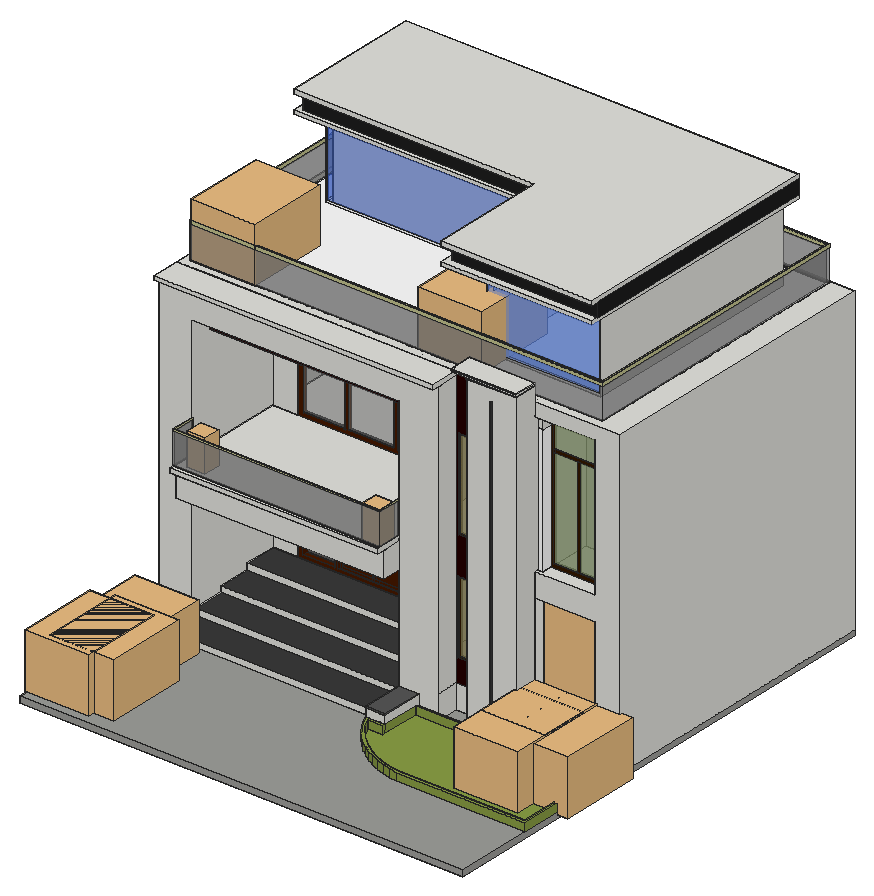
# SketchUp Ruby script. Lengths in inches.
U = 1.inch
M = Sketchup.active_model
def pt(a) = Geom::Point3d.new(a.map { |v| v * U })
def face(e, loops, mat)
  f = e.add_face(loops[0].map { |a| pt(a) })
  loops[1..].each { |l| e.add_face(l.map { |a| pt(a) }).erase! }
  f.material = f.back_material = mat if mat
  f
end
# faces: each face lists its corners as indices into pts; further lists are holes
def faces(e, pts, list, mat = nil) = list.each { |f| face(e, (f[0].is_a?(Array) ? f : [f]).map { |l| l.map { |i| pts[i] } }, mat) }
# xy, xz, yz: faces in a plane at the given z, y or x. An outline is a flat list of corners, or four numbers for a rectangle; further outlines are holes
def ring(l) = l.size == 4 ? [[l[0], l[1]], [l[2], l[1]], [l[2], l[3]], [l[0], l[3]]] : l.each_slice(2).to_a
def flat(e, list, mat, &to3) = list.each { |f| face(e, (f[0].is_a?(Array) ? f : [f]).map { |l| ring(l).map { |u, v| to3.(u, v) } }, mat) }
def xy(e, z, list, mat = nil) = flat(e, list, mat) { |x, y| [x, y, z] }
def xz(e, y, list, mat = nil) = flat(e, list, mat) { |x, z| [x, y, z] }
def yz(e, x, list, mat = nil) = flat(e, list, mat) { |y, z| [x, y, z] }
def lines(e, pts, list) = list.each { |a, b| e.add_line(pt(pts[a]), pt(pts[b])) }
# prism: a flat outline (further loops are holes) pulled along v
def prism(e, loops, v, mat = nil)
  f = face(e, loops, mat); d = Geom::Vector3d.new(v.map { |x| x * U })
  f.pushpull(f.normal.samedirection?(d) ? d.length : -d.length)
end
def box(e, o, s, mat = nil) = prism(e, [[o, [o[0] + s[0], o[1], o[2]], [o[0] + s[0], o[1] + s[1], o[2]], [o[0], o[1] + s[1], o[2]]]], [0, 0, s[2]], mat)
def at(x, y, z, deg = 0) = Geom::Transformation.translation(pt([x, y, z])) * Geom::Transformation.rotation(ORIGIN, Z_AXIS, deg.degrees)
def axes(o, x, y, z) = Geom::Transformation.new([*x, 0, *y, 0, *z, 0, *pt(o).to_a, 1])
def part(name) = M.definitions.add(name)
# library, detail: a bought-in or finely detailed component or shape, given as its bounding box
def library(name, o, s) = part(name).tap { |d| box(d.entities, o, s) }
def detail(e, o, s) = box(e.add_group.entities, o, s)
def put(e, d, t, mat = nil) = e.add_instance(d, t).tap { |i| i.material = mat if mat }
def group(e, t, mat = nil) = e.add_group.tap { |g| g.transformation = t; g.material = mat if mat }.entities
root = M.entities
M.materials.add("[Color A08]").color = [37, 0, 0]
M.materials.add("[Color B08]").color = [71, 25, 0]
M.materials.add("[Color B08]1").color = [52, 25, 0]
M.materials.add("[Color M00]").color = [255, 255, 255]
M.materials.add("[Color M06]").color = [86, 86, 86]
M.materials.add("[Color M07]").color = [58, 58, 58]
M.materials.add("[Color M08]").color = [30, 30, 30]
M.materials.add("[Concrete Block 8x8 Gray]").color = [157, 158, 154]
M.materials.add("[Grass Light Green]").color = [138, 158, 69]
M.materials.add("[Metal Corrugated Shiny]").color = [193, 193, 151]
M.materials.add("[Metal Corrugated Shiny]1").color = [193, 193, 141]
M.materials.add("[Translucent Glass Corrugated]").color = [141, 132, 85]
M.materials["[Translucent Glass Corrugated]"].alpha = 0.8
M.materials.add("[Translucent Glass Corrugated]1").color = [141, 158, 115]
M.materials["[Translucent Glass Corrugated]1"].alpha = 0.8
M.materials.add("[Translucent Glass Gray]").color = [128, 128, 128]
M.materials["[Translucent Glass Gray]"].alpha = 0.5
M.materials.add("[Translucent Glass Safety]").color = [100, 143, 244]
M.materials["[Translucent Glass Safety]"].alpha = 0.5
M.materials.add("[Translucent Glass Safety]1").color = [69, 115, 244]
M.materials["[Translucent Glass Safety]1"].alpha = 0.5
c1 = library("ARTIFICIAL PLANTS",[20.77,3.52,-2.22],[96.42,122.82,82.56])
c2 = library("Plant",[12.07,-11.84,0],[27.54,27.97,38.79])
c3 = part("Group\#3")
xy(c3.entities,0,[[0,0,37.8125,3.1875]],"[Color B08]1")
xy(c3.entities,2.15,[[2.15,0,35.67,0.6875],[2.15,0.6875,35.67,3.1875]],"[Color B08]1")
xy(c3.entities,107.17,[[2.15,0,35.67,0.6875],[2.15,0.6875,35.67,3.1875]],"[Color B08]1")
xy(c3.entities,109.3125,[[0,0,37.8125,3.1875]],"[Color B08]1")
xz(c3.entities,0,[[[0,0,37.8125,109.3125],[2.15,2.15,35.67,107.17]]],"[Color B08]1")
xz(c3.entities,0.6875,[[2.15,2.15,35.67,107.17]],"[Translucent Glass Corrugated]")
xz(c3.entities,3.1875,[[[0,0,37.8125,109.3125],[2.15,2.15,35.67,107.17]]],"[Color B08]1")
yz(c3.entities,0,[[0,0,3.1875,109.3125]],"[Color B08]1")
yz(c3.entities,2.15,[[0,2.15,0.6875,107.17],[0.6875,2.15,3.1875,107.17]],"[Color B08]1")
yz(c3.entities,35.67,[[0,2.15,0.6875,107.17],[0.6875,2.15,3.1875,107.17]],"[Color B08]1")
yz(c3.entities,37.8125,[[0,0,3.1875,109.3125]],"[Color B08]1")
c4 = library("Group\#4",[0,0,0],[79.3125,7.3125,150.8125])
xy(root,0,[[0,0,667.75,739.0625]])
xy(root,9,[[24.41,199.0625,48.8125,262.25],[362.125,199.0625,391.71,262.25],[0,262.25,48.8125,295.75],[362.125,262.25,421.3,295.75],[[0,295.75,0,739.0625,667.75,739.0625,667.75,295.75,539.36,295.75,539.36,301.75,547.4375,301.75,547.4375,730.0625,366.0625,730.0625,366.0625,415.1875,48.8125,415.1875,48.8125,295.75],[48.8125,421.1875,362.125,730.0625],[553.4375,301.75,630.8125,730.0625]],
  [362.125,295.75,463.53,301.75],[362.125,301.75,366.0625,415.1875],[366.0625,301.75,547.4375,730.0625],[553.4375,301.75,630.8125,730.0625],[48.8125,421.1875,362.125,730.0625]])
xy(root,9,[[500.61,259.1875,502.54,262.25]],"[Color M07]")
xy(root,9,[[0,0,667.75,0,667.75,117.6,474.66,117.6,462.59,119.14,450.71,121.76,439.11,125.45,427.9,130.18,417.16,135.91,406.99,142.59,397.47,150.16,388.68,158.57,380.68,167.75,373.55,177.61,367.35,188.07,362.125,199.0625,362.125,415.1875,48.8125,415.1875,48.8125,199.0625,24.41,199.0625,24.41,262.25,0,262.25],[391.71,259.1875,500.61,259.1875,500.61,262.25,463.53,262.25,463.53,295.75,421.3,295.75,421.3,262.25,391.71,262.25]],"[Concrete Block 8x8 Gray]")
xy(root,9,[[474.66,117.6,462.59,119.14,450.71,121.76,439.11,125.45,427.9,130.18,417.16,135.91,406.99,142.59,397.47,150.16,388.68,158.57,380.68,167.75,373.55,177.61,367.35,188.07,362.125,199.0625,391.71,199.0625,391.71,195.14,368.33,195.14,370.82,189.92,376.84,179.76,383.76,170.1875,391.52,161.28,400.05,153.12,409.3,145.77,419.17,139.29,429.59,133.73,440.47,129.14,451.73,125.55,463.26,123.01,474.91,121.53,663.83,121.53,663.83,292.2,539.36,292.2,539.36,295.75,667.75,295.75,667.75,117.6],[474.91,121.53,663.83,121.53,663.83,292.2,541.86,292.2,541.86,256.08,391.71,256.08,391.71,195.14,368.33,195.14,370.82,189.92,376.84,179.76,383.76,170.1875,391.52,161.28,400.05,153.12,409.3,145.77,419.17,139.29,429.59,133.73,440.47,129.14,451.73,125.55,463.26,123.01],[391.71,256.08,391.71,259.1875,502.54,259.1875,502.54,262.25,541.86,262.25,541.86,256.08]],"[Grass Light Green]")
xy(root,21,[[474.66,117.6,667.75,117.6,667.75,295.75,539.36,295.75,539.36,262.25,502.54,262.25,502.54,259.1875,391.71,259.1875,391.71,256.08,541.86,256.08,541.86,292.2,663.83,292.2,663.83,121.53,474.91,121.53,463.26,123.01,451.73,125.55,440.47,129.14,429.59,133.73,419.17,139.29,409.3,145.77,400.05,153.12,391.52,161.28,383.76,170.1875,376.84,179.76,370.82,189.92,368.33,195.14,391.71,195.14,391.71,199.0625,362.125,199.0625,367.35,188.07,373.55,177.61,380.68,167.75,388.68,158.57,397.47,150.16,406.99,142.59,417.16,135.91,427.9,130.18,439.11,125.45,450.71,121.76,462.59,119.14]],"[Grass Light Green]")
xy(root,33,[[24.41,199.0625,48.8125,262.25],[362.125,199.0625,391.71,262.25]])
xy(root,35,[[362.125,199.0625,391.71,262.25]],"[Color M06]")
xy(root,35.25,[[24.41,199.0625,48.8125,262.25]],"[Color M06]")
xy(root,45,[[547.4375,295.75,547.4375,303.1875,553.4375,303.1875,553.4375,301.75,553.875,301.75,553.875,295.75],[553.875,295.75,630.8125,301.75],[553.4375,301.75,553.875,730.0625],[547.4375,303.1875,553.4375,730.0625],[86.78,415.1875,319.35,421.1875]])
xy(root,79.74,[[424.46,295.75,460.15,301.75]])
xy(root,182,[[86.78,415.1875,319.35,421.1875]])
xy(root,190.99,[[424.46,295.75,460.15,301.75]])
xy(root,191.8125,[[48.8125,232.8125,362.125,415.1875]])
xy(root,201,[[547.4375,295.75,547.4375,303.1875,553.4375,303.1875,553.4375,301.75,553.875,301.75,553.875,295.75],[362.125,301.75,366.0625,415.1875],[553.4375,301.75,553.875,381.8125],[547.4375,303.1875,553.4375,730.0625]])
xy(root,201,[[553.875,295.75,630.8125,381.8125]],"[Color M00]")
xy(root,211.75,[[553.4375,381.8125,630.8125,730.0625]])
xy(root,227.875,[[48.8125,421.1875,362.125,730.0625]])
xy(root,230.8125,[[48.8125,222.0625,362.125,232.8125],[48.8125,232.8125,48.8125,415.1875,86.78,415.1875,86.78,421.1875,319.35,421.1875,319.35,415.1875,362.125,415.1875,362.125,232.8125]])
xy(root,231,[[366.0625,301.75,547.4375,730.0625]])
xy(root,237,[[48.8125,222.0625,362.125,226.625],[48.8125,226.625,48.8125,262.25,50.625,262.25,50.625,228.625,360.31,228.625,360.31,262.25,362.125,262.25,362.125,226.625],[50.625,228.625,360.31,228.625,360.31,262.25,362.125,262.25,362.125,415.1875,319.35,415.1875,319.35,421.1875,86.78,421.1875,86.78,415.1875,48.8125,415.1875,48.8125,262.25,50.625,262.25],[539.36,295.75,539.36,301.75,547.4375,301.75,547.4375,316.75,630.8125,316.75,630.8125,295.75],[362.125,301.75,366.0625,415.1875],
  [366.0625,301.75,547.4375,730.0625],[547.4375,320.84,630.8125,381.8125],[553.4375,381.8125,630.8125,730.0625],[48.8125,421.1875,362.125,730.0625]])
xy(root,237,[[547.4375,316.75,630.8125,320.84]],"[Color B08]1")
xy(root,242.04,[[551.26,316.75,587.21,318.46],[587.21,316.75,590.4375,318.46],[590.4375,316.75,626.99,318.46],[551.26,318.46,587.21,320.84],[587.21,318.46,590.4375,320.84],
  [590.4375,318.46,626.99,320.84]],"[Color B08]1")
xy(root,246,[[425.47,295.75,460.78,301.75]])
xy(root,285,[[48.8125,226.625,48.8125,262.25,50.625,262.25,50.625,228.625,360.31,228.625,360.31,262.25,362.125,262.25,362.125,226.625]])
xy(root,287.0625,[[48.8125,226.625,362.125,226.625,362.125,262.25,360.31,262.25,360.31,228.625,50.625,228.625,50.625,262.25,48.8125,262.25]],"[Metal Corrugated Shiny]1")
xy(root,374,[[86.78,415.1875,319.35,421.1875]])
xy(root,384.44,[[425.47,295.75,460.78,301.75]])
xy(root,393,[[362.125,301.75,366.0625,415.1875]])
xy(root,393,[[48.8125,295.75,362.125,415.1875]],"[Color M07]")
xy(root,419.72,[[48.8125,262.25,362.125,295.75]])
xy(root,429,[[366.0625,301.75,547.375,301.75,547.375,336.875,547.4375,336.875,547.4375,730.0625,366.0625,730.0625],[547.375,301.75,547.4375,332.6875],[547.4375,301.75,547.875,332.6875],[547.375,332.6875,547.4375,336.875],[547.4375,381.8125,553.4375,730.0625],
  [553.4375,381.8125,630.8125,730.0625]])
xy(root,429,[[547.4375,332.6875,630.8125,381.8125]],"[Color M00]")
xy(root,441.39,[[551.26,316.75,626.99,318.46],[551.26,318.46,626.99,320.84]],"[Color B08]1")
xy(root,446.4375,[[539.36,295.75,547.875,301.75],[547.875,295.75,630.8125,316.75],[366.0625,301.75,366.0625,730.0625,630.8125,730.0625,630.8125,336.875,547.375,336.875,547.375,301.75],[547.375,301.75,547.875,301.75,547.875,316.75,547.4375,316.75,547.4375,320.84,547.875,320.84,547.875,332.6875,630.8125,332.6875,630.8125,336.875,547.375,336.875],[547.4375,316.75,547.875,320.84],
  [547.875,320.84,630.8125,332.6875]])
xy(root,446.4375,[[547.875,316.75,630.8125,320.84]],"[Color B08]1")
xy(root,460.0625,[[0,252.125,421.3,262.25],[0,262.25,421.3,295.75]])
xy(root,466.375,[[0,252.125,421.3,295.75],[[0,295.75,667.75,739.0625],[9.3125,307.9375,632.75,735.0625]],[[9.3125,307.9375,632.75,735.0625],[11.3125,309.9375,630.75,733.0625]],[[420.125,354.47,420.125,517.125,48.125,517.125,48.125,696.4375,593.125,696.4375,593.125,354.47],[426.125,360.47,587.125,360.47,587.125,690.4375,54.125,690.4375,54.125,523.125,426.125,523.125]],[426.125,360.47,587.125,360.47,587.125,690.4375,54.125,690.4375,54.125,523.125,426.125,523.125]])
xy(root,466.375,[[[11.3125,309.9375,630.75,733.0625],[420.125,354.47,593.125,354.47,593.125,696.4375,48.125,696.4375,48.125,517.125,420.125,517.125]]],"[Color M00]")
xy(root,467.84,[[500.61,259.1875,502.54,262.25]],"[Color M07]")
xy(root,486.125,[[463.53,261.625,539.36,262.25],[463.53,262.25,539.36,295.75]])
xy(root,488.1875,[[442.91,260.8125,463.53,295.75],[463.53,260.8125,539.36,261.625],[463.53,261.625,539.36,295.75]])
xy(root,490.625,[[441.16,260.0625,442.91,295.75],[442.91,260.0625,539.36,260.8125],[442.91,260.8125,539.36,295.75]])
xy(root,492.0625,[[441.16,260.0625,539.36,295.75]])
xy(root,514.375,[[[9.3125,307.9375,632.75,735.0625],[11.3125,309.9375,630.75,733.0625]]])
xy(root,519.75,[[[9.3125,307.9375,632.75,735.0625],[11.3125,309.9375,630.75,733.0625]]],"[Metal Corrugated Shiny]1")
xy(root,580.375,[[426.125,360.47,426.125,523.125,54.125,523.125,54.125,690.4375,587.125,690.4375,587.125,360.47]])
xy(root,586.375,[[381.75,315.41,381.75,492.1875,18.75,492.1875,18.75,704.25,48.125,704.25,48.125,517.125,420.125,517.125,420.125,354.47,593.125,354.47,593.125,696.4375,63,696.4375,63,704.25,610.625,704.25,610.625,315.41],[420.125,354.47,426.125,508.125],[426.125,354.47,593.125,360.47],[426.125,360.47,426.125,523.125,54.125,523.125,54.125,690.4375,587.125,690.4375,587.125,360.47],[587.125,360.47,593.125,690.4375],
  [420.125,508.125,426.125,508.125,426.125,523.125,54.125,523.125,54.125,517.125,420.125,517.125],[48.125,517.125,54.125,696.4375],[54.125,690.4375,63,696.4375],[63,690.4375,593.125,696.4375],[48.125,696.4375,54.125,704.25],
  [54.125,696.4375,63,704.25]])
xy(root,591.75,[[381.75,315.41,610.625,315.41,610.625,326.35,390.1875,326.35,390.1875,492.1875,381.75,492.1875],[390.1875,326.35,610.625,326.35,610.625,704.25,63,704.25,63,696.4375,593.125,696.4375,593.125,354.47,420.125,354.47,420.125,517.125,48.125,517.125,48.125,704.25,28.5625,704.25,28.5625,498.4375,390.1875,498.4375],[420.125,354.47,593.125,354.47,593.125,696.4375,63,696.4375,63,704.25,48.125,704.25,48.125,517.125,420.125,517.125],[18.75,492.1875,390.1875,492.1875,390.1875,498.4375,28.5625,498.4375,28.5625,704.25,18.75,704.25]])
xy(root,612.75,[[381.75,315.41,381.75,492.1875,18.75,492.1875,18.75,704.25,28.5625,704.25,28.5625,498.4375,390.1875,498.4375,390.1875,326.35,610.625,326.35,610.625,315.41]])
xy(root,619.25,[[381.75,315.41,610.625,315.41,610.625,704.25,18.75,704.25,18.75,492.1875,381.75,492.1875]])
xz(root,0,[[0,0,667.75,9]],"[Concrete Block 8x8 Gray]")
xz(root,117.6,[[474.66,9,667.75,21]],"[Grass Light Green]")
xz(root,121.53,[[474.91,9,663.83,21]],"[Grass Light Green]")
xz(root,195.14,[[368.33,9,391.71,21]],"[Grass Light Green]")
xz(root,199.0625,[[24.41,9,48.8125,33],[362.125,21,391.71,33]])
xz(root,199.0625,[[24.41,33,48.8125,35.25],[362.125,33,391.71,35]],"[Color M06]")
xz(root,199.0625,[[362.125,9,391.71,21]],"[Grass Light Green]")
xz(root,222.0625,[[48.8125,230.8125,362.125,237]])
xz(root,226.625,[[48.8125,285,362.125,287.0625]],"[Metal Corrugated Shiny]1")
xz(root,226.625,[[48.8125,237,362.125,285]],"[Translucent Glass Gray]")
xz(root,228.625,[[50.625,285,360.31,287.0625]],"[Metal Corrugated Shiny]1")
xz(root,228.625,[[50.625,237,360.31,285]],"[Translucent Glass Gray]")
xz(root,232.8125,[[48.8125,191.8125,362.125,230.8125]])
xz(root,252.125,[[0,460.0625,421.3,466.375]])
xz(root,256.08,[[391.71,9,541.86,21]],"[Grass Light Green]")
xz(root,259.1875,[[500.61,9,502.54,21],[500.61,21,502.54,467.84]],"[Color M07]")
xz(root,259.1875,[[391.71,9,500.61,21]],"[Grass Light Green]")
xz(root,260.0625,[[441.16,490.625,539.36,492.0625]])
xz(root,260.8125,[[442.91,488.1875,539.36,490.625]])
xz(root,261.625,[[463.53,486.125,539.36,488.1875]])
xz(root,262.25,[[0,9,24.41,9,24.41,35.25,48.8125,35.25,48.8125,419.72,362.125,419.72,362.125,35,391.71,35,391.71,9,421.3,9,421.3,460.0625,0,460.0625],[24.41,9,48.8125,33],[362.125,9,391.71,33],[463.53,9,500.61,9,500.61,467.84,502.54,467.84,502.54,21,539.36,21,539.36,486.125,463.53,486.125],[24.41,33,48.8125,35.25],
  [362.125,33,391.71,35],[48.8125,237,50.625,285],[360.31,237,362.125,285],[48.8125,285,50.625,287.0625],[360.31,285,362.125,287.0625]])
xz(root,262.25,[[500.61,9,502.54,467.84]],"[Color M07]")
xz(root,292.2,[[541.86,9,663.83,21]],"[Grass Light Green]")
xz(root,295.75,[[421.3,9,463.53,45],[539.36,21,667.75,21,667.75,466.375,539.36,466.375,539.36,446.4375,630.8125,446.4375,630.8125,237,539.36,237,539.36,201,630.8125,201,630.8125,45,539.36,45],[539.36,45,553.875,201],[48.8125,419.72,362.125,460.0625],[0,460.0625,48.8125,466.375],
  [48.8125,460.0625,362.125,466.375],[362.125,460.0625,421.3,466.375],[463.53,466.375,539.36,486.125],[463.53,486.125,539.36,488.1875],[442.91,488.1875,539.36,490.625],
  [441.16,490.625,539.36,492.0625]])
xz(root,295.75,[[[421.3,45,463.53,466.375],[425.47,246,460.78,384.44],[424.46,79.74,460.15,190.99]],[48.8125,393,362.125,419.72]],"[Color A08]")
xz(root,301.75,[[[366.0625,9,463.53,231],[424.46,79.74,460.15,190.99]],[463.53,9,539.36,45],[539.36,9,547.4375,45],[553.4375,9,630.8125,45],[463.53,45,539.36,201],
  [539.36,45,547.4375,201],[553.4375,45,553.875,201],[362.125,201,366.0625,237],[463.53,201,539.36,231],[539.36,201,547.4375,231],
  [366.0625,231,463.53,237],[463.53,231,539.36,237],[539.36,231,547.4375,237],[[366.0625,237,539.36,429],[425.47,246,460.78,384.44]],[366.0625,429,539.36,446.4375],
  [539.36,429,547.875,446.4375],[463.53,446.4375,539.36,460.0625]])
xz(root,301.75,[[539.36,237,547.4375,429]],"[Color M00]")
xz(root,303.1875,[[547.4375,45,553.4375,201]])
xz(root,307.9375,[[9.3125,514.375,632.75,519.75]],"[Metal Corrugated Shiny]1")
xz(root,307.9375,[[9.3125,466.375,632.75,514.375]],"[Translucent Glass Gray]")
xz(root,309.9375,[[11.3125,514.375,630.75,519.75]],"[Metal Corrugated Shiny]1")
xz(root,309.9375,[[11.3125,466.375,630.75,514.375]],"[Translucent Glass Gray]")
xz(root,315.41,[[381.75,586.375,610.625,591.75],[381.75,612.75,610.625,619.25]])
xz(root,316.75,[[[547.4375,237,630.8125,446.4375],[551.26,242.04,626.99,441.39]]],"[Color B08]1")
xz(root,318.46,[[587.21,242.04,590.4375,391.43],[551.26,391.43,626.99,396.74]],"[Color B08]1")
xz(root,318.46,[[551.26,242.04,587.21,391.43],[590.4375,242.04,626.99,391.43],[551.26,396.74,626.99,441.39]],"[Translucent Glass Corrugated]1")
xz(root,320.84,[[[547.4375,237,630.8125,446.4375],[551.26,242.04,626.99,441.39]]],"[Color B08]1")
xz(root,326.35,[[390.1875,591.75,610.625,612.75]],"[Color M08]")
xz(root,332.6875,[[547.875,429,630.8125,446.4375]])
xz(root,354.47,[[420.125,586.375,426.125,591.75],[426.125,586.375,593.125,591.75]])
xz(root,354.47,[[[420.125,466.375,593.125,586.375],[422.51,468.76,590.74,583.99]]],"[Color M00]")
xz(root,354.47,[[422.51,468.76,590.74,583.99]],"[Translucent Glass Safety]")
xz(root,360.47,[[426.125,580.375,587.125,586.375]])
xz(root,360.47,[[426.125,466.375,587.125,580.375]],"[Translucent Glass Safety]")
xz(root,381.8125,[[553.4375,201,630.8125,211.75],[553.4375,211.75,630.8125,237],[547.4375,237,630.8125,429]])
xz(root,415.1875,[[48.8125,9,362.125,45],[362.125,9,366.0625,45],[48.8125,45,86.78,45,86.78,182,319.35,182,319.35,45,362.125,45,362.125,191.8125,48.8125,191.8125],[362.125,45,366.0625,201],[48.8125,230.8125,86.78,237],
  [319.35,230.8125,362.125,237],[48.8125,237,86.78,237,86.78,374,319.35,374,319.35,237,362.125,237,362.125,393,48.8125,393],[362.125,237,366.0625,393]])
xz(root,421.1875,[[48.8125,9,362.125,45],[48.8125,45,48.8125,201,362.125,201,362.125,45,319.35,45,319.35,182,86.78,182,86.78,45],[48.8125,201,362.125,227.875],[48.8125,227.875,86.78,237],[86.78,227.875,319.35,230.8125],
  [319.35,227.875,328.9375,237],[328.9375,227.875,350.5,237],[350.5,227.875,362.125,237],[86.78,230.8125,319.35,237],[48.8125,237,48.8125,393,362.125,393,362.125,237,319.35,237,319.35,374,86.78,374,86.78,237],
  [48.8125,393,362.125,429]])
xz(root,492.1875,[[18.75,586.375,381.75,591.75],[18.75,612.75,381.75,619.25]])
xz(root,498.4375,[[28.5625,591.75,390.1875,612.75]],"[Color M08]")
xz(root,517.125,[[48.125,586.375,54.125,591.75],[54.125,586.375,420.125,591.75]])
xz(root,517.125,[[[48.125,466.375,420.125,586.375],[50.82,469.07,417.43,583.68]]],"[Color M00]")
xz(root,517.125,[[50.82,469.07,417.43,583.68]],"[Translucent Glass Safety]1")
xz(root,523.125,[[54.125,466.375,426.125,580.375],[54.125,580.375,426.125,586.375]])
xz(root,690.4375,[[54.125,466.375,587.125,580.375],[54.125,580.375,63,586.375],[63,580.375,587.125,586.375]])
xz(root,696.4375,[[48.125,466.375,593.125,586.375],[63,586.375,593.125,591.75]])
xz(root,704.25,[[18.75,586.375,610.625,591.75],[18.75,612.75,610.625,619.25]])
xz(root,704.25,[[28.5625,591.75,610.625,612.75]],"[Color M08]")
xz(root,730.0625,[[48.8125,9,362.125,45],[366.0625,9,547.4375,45],[553.4375,9,630.8125,45],[48.8125,45,362.125,201],[366.0625,45,547.4375,201],
  [547.4375,45,553.4375,201],[553.4375,45,553.875,201],[553.875,45,630.8125,201],[48.8125,201,362.125,227.875],[366.0625,201,547.4375,231],
  [547.4375,201,553.4375,429],[553.4375,201,630.8125,211.75],[553.4375,211.75,561.3125,237],[561.3125,211.75,573.8125,237],[573.8125,211.75,630.8125,237],
  [48.8125,227.875,362.125,237],[366.0625,231,547.4375,237],[48.8125,237,362.125,393],[366.0625,237,547.4375,393],[553.4375,237,630.8125,393],
  [48.8125,393,362.125,429],[366.0625,393,547.4375,429],[553.4375,393,630.8125,429],[366.0625,429,547.4375,446.4375],[547.4375,429,553.4375,446.4375],
  [553.4375,429,630.8125,446.4375]])
xz(root,733.0625,[[11.3125,514.375,630.75,519.75]],"[Metal Corrugated Shiny]1")
xz(root,733.0625,[[11.3125,466.375,630.75,514.375]],"[Translucent Glass Gray]")
xz(root,735.0625,[[9.3125,514.375,632.75,519.75]],"[Metal Corrugated Shiny]1")
xz(root,735.0625,[[9.3125,466.375,632.75,514.375]],"[Translucent Glass Gray]")
xz(root,739.0625,[[0,9,667.75,466.375]])
xz(root,739.0625,[[0,0,667.75,9]],"[Concrete Block 8x8 Gray]")
yz(root,0,[[262.25,9,262.25,460.0625,295.75,460.0625,295.75,466.375,739.0625,466.375,739.0625,9],[252.125,460.0625,295.75,466.375]])
yz(root,0,[[0,0,739.0625,9]],"[Concrete Block 8x8 Gray]")
yz(root,9.3125,[[307.9375,514.375,735.0625,519.75]],"[Metal Corrugated Shiny]1")
yz(root,9.3125,[[307.9375,466.375,735.0625,514.375]],"[Translucent Glass Gray]")
yz(root,11.3125,[[309.9375,514.375,733.0625,519.75]],"[Metal Corrugated Shiny]1")
yz(root,11.3125,[[309.9375,466.375,733.0625,514.375]],"[Translucent Glass Gray]")
yz(root,18.75,[[492.1875,586.375,704.25,591.75],[492.1875,612.75,704.25,619.25]])
yz(root,24.41,[[199.0625,9,262.25,33]])
yz(root,24.41,[[199.0625,33,262.25,35.25]],"[Color M06]")
yz(root,28.5625,[[498.4375,591.75,704.25,612.75]],"[Color M08]")
yz(root,48.125,[[517.125,586.375,696.4375,591.75]])
yz(root,48.125,[[[517.125,466.375,696.4375,586.375],[518.72,467.97,694.84,584.78]]],"[Color M00]")
yz(root,48.125,[[518.72,467.97,694.84,584.78]],"[Translucent Glass Safety]1")
yz(root,48.8125,[[199.0625,9,262.25,33],[262.25,9,415.1875,191.8125],[421.1875,9,730.0625,45],[421.1875,45,730.0625,201],[232.8125,191.8125,262.25,230.8125],
  [262.25,191.8125,295.75,230.8125],[421.1875,201,730.0625,227.875],[421.1875,227.875,730.0625,237],[222.0625,230.8125,262.25,237],[262.25,230.8125,295.75,237],
  [295.75,230.8125,415.1875,237],[262.25,237,415.1875,237,415.1875,393,295.75,393,295.75,419.72,262.25,419.72],[421.1875,237,730.0625,393],[421.1875,393,730.0625,429]])
yz(root,48.8125,[[199.0625,33,262.25,35.25]],"[Color M06]")
yz(root,48.8125,[[226.625,285,262.25,287.0625]],"[Metal Corrugated Shiny]1")
yz(root,48.8125,[[226.625,237,262.25,285]],"[Translucent Glass Gray]")
yz(root,50.625,[[228.625,285,262.25,287.0625]],"[Metal Corrugated Shiny]1")
yz(root,50.625,[[228.625,237,262.25,285]],"[Translucent Glass Gray]")
yz(root,54.125,[[523.125,466.375,690.4375,580.375],[523.125,580.375,690.4375,586.375]])
yz(root,86.78,[[415.1875,45,421.1875,182],[415.1875,230.8125,421.1875,237],[415.1875,237,421.1875,374]])
yz(root,319.35,[[415.1875,45,421.1875,182],[415.1875,230.8125,421.1875,237],[415.1875,237,421.1875,374]])
yz(root,360.31,[[228.625,285,262.25,287.0625]],"[Metal Corrugated Shiny]1")
yz(root,360.31,[[228.625,237,262.25,285]],"[Translucent Glass Gray]")
yz(root,362.125,[[199.0625,9,262.25,33],[262.25,9,415.1875,191.8125],[421.1875,9,730.0625,45],[421.1875,45,730.0625,201],[232.8125,191.8125,262.25,230.8125],
  [262.25,191.8125,295.75,230.8125],[295.75,191.8125,301.75,230.8125],[301.75,191.8125,415.1875,201],[421.1875,201,730.0625,227.875],[421.1875,227.875,730.0625,237],
  [222.0625,230.8125,262.25,237],[262.25,230.8125,295.75,237],[295.75,230.8125,301.75,237],[301.75,230.8125,415.1875,237],[262.25,237,262.25,419.72,295.75,419.72,295.75,393,415.1875,393,415.1875,237],
  [421.1875,237,730.0625,393],[421.1875,393,730.0625,429]])
yz(root,362.125,[[199.0625,33,262.25,35]],"[Color M06]")
yz(root,362.125,[[226.625,285,262.25,287.0625]],"[Metal Corrugated Shiny]1")
yz(root,362.125,[[226.625,237,262.25,285]],"[Translucent Glass Gray]")
yz(root,366.0625,[[301.75,9,415.1875,45],[415.1875,9,730.0625,45],[301.75,45,415.1875,201],[415.1875,45,730.0625,201],[301.75,201,415.1875,231],
  [415.1875,201,730.0625,231],[301.75,231,415.1875,237],[415.1875,231,730.0625,237],[301.75,237,415.1875,393],[415.1875,237,730.0625,393],
  [301.75,393,415.1875,429],[415.1875,393,730.0625,429],[301.75,429,415.1875,446.4375],[415.1875,429,730.0625,446.4375]])
yz(root,381.75,[[315.41,586.375,492.1875,591.75],[315.41,612.75,492.1875,619.25]])
yz(root,390.1875,[[326.35,591.75,498.4375,612.75]],"[Color M08]")
yz(root,391.71,[[259.1875,9,262.25,9,262.25,33,199.0625,33,199.0625,21,259.1875,21]])
yz(root,391.71,[[199.0625,33,262.25,35]],"[Color M06]")
yz(root,391.71,[[195.14,9,199.0625,21],[199.0625,9,256.08,21],[256.08,9,259.1875,21]],"[Grass Light Green]")
yz(root,420.125,[[354.47,586.375,508.125,591.75],[508.125,586.375,517.125,591.75]])
yz(root,420.125,[[[354.47,466.375,517.125,586.375],[356.23,468.13,515.37,584.62]]],"[Color M00]")
yz(root,420.125,[[356.23,468.13,515.37,584.62]],"[Translucent Glass Safety]1")
yz(root,421.3,[[262.25,9,295.75,45],[262.25,45,295.75,460.0625],[252.125,460.0625,295.75,466.375]])
yz(root,424.46,[[295.75,79.74,301.75,190.99]])
yz(root,425.47,[[295.75,246,301.75,384.44]])
yz(root,426.125,[[360.47,466.375,523.125,580.375],[360.47,580.375,523.125,586.375]])
yz(root,441.16,[[260.0625,490.625,295.75,492.0625]])
yz(root,442.91,[[260.8125,488.1875,295.75,490.625]])
yz(root,460.15,[[295.75,79.74,301.75,190.99]])
yz(root,460.78,[[295.75,246,301.75,384.44]])
yz(root,463.53,[[262.25,9,295.75,486.125],[295.75,9,301.75,45],[261.625,486.125,295.75,488.1875]])
yz(root,500.61,[[259.1875,9,262.25,467.84]],"[Color M07]")
yz(root,502.54,[[259.1875,21,262.25,467.84]],"[Color M07]")
yz(root,502.54,[[259.1875,9,262.25,21]],"[Grass Light Green]")
yz(root,539.36,[[295.75,9,301.75,45],[262.25,21,295.75,21,295.75,237,301.75,237,301.75,446.4375,295.75,446.4375,295.75,486.125,262.25,486.125],[295.75,45,301.75,201],[295.75,201,301.75,237],[295.75,446.4375,301.75,460.0625],
  [261.625,486.125,295.75,488.1875],[260.8125,488.1875,295.75,490.625],[260.0625,490.625,295.75,492.0625]])
yz(root,539.36,[[292.2,9,295.75,21]],"[Grass Light Green]")
yz(root,541.86,[[256.08,9,292.2,21]],"[Grass Light Green]")
yz(root,547.4375,[[301.75,9,730.0625,45],[301.75,45,303.1875,201],[303.1875,45,730.0625,201],[301.75,201,730.0625,231],[301.75,231,381.8125,237],
  [381.8125,231,730.0625,237],[381.8125,237,730.0625,393],[381.8125,393,730.0625,429]])
yz(root,547.4375,[[316.75,237,320.84,429],[316.75,429,320.84,446.4375]],"[Color B08]1")
yz(root,547.4375,[[301.75,237,316.75,429],[320.84,237,381.8125,429]],"[Color M00]")
yz(root,547.875,[[301.75,429,332.6875,446.4375]])
yz(root,551.26,[[316.75,242.04,318.46,391.43],[318.46,242.04,320.84,391.43],[316.75,391.43,318.46,396.74],[318.46,391.43,320.84,396.74],[316.75,396.74,318.46,441.39],
  [318.46,396.74,320.84,441.39]],"[Color B08]1")
yz(root,553.4375,[[301.75,9,730.0625,45],[301.75,45,303.1875,201],[303.1875,45,730.0625,201],[381.8125,201,730.0625,211.75],[381.8125,211.75,730.0625,237]])
yz(root,553.875,[[295.75,45,301.75,201]])
yz(root,587.125,[[360.47,580.375,690.4375,586.375]])
yz(root,587.125,[[360.47,466.375,690.4375,580.375]],"[Translucent Glass Safety]")
yz(root,593.125,[[354.47,466.375,696.4375,586.375],[354.47,586.375,360.47,591.75],[360.47,586.375,690.4375,591.75],[690.4375,586.375,696.4375,591.75]])
yz(root,610.625,[[315.41,586.375,704.25,591.75],[315.41,612.75,704.25,619.25]])
yz(root,610.625,[[326.35,591.75,704.25,612.75]],"[Color M08]")
yz(root,626.99,[[316.75,242.04,318.46,391.43],[318.46,242.04,320.84,391.43],[316.75,391.43,318.46,396.74],[318.46,391.43,320.84,396.74],[316.75,396.74,318.46,441.39],
  [318.46,396.74,320.84,441.39]],"[Color B08]1")
yz(root,630.75,[[309.9375,514.375,733.0625,519.75]],"[Metal Corrugated Shiny]1")
yz(root,630.75,[[309.9375,466.375,733.0625,514.375]],"[Translucent Glass Gray]")
yz(root,630.8125,[[301.75,9,730.0625,45],[295.75,45,730.0625,201],[381.8125,201,730.0625,211.75],[381.8125,211.75,730.0625,237],[295.75,237,316.75,446.4375],
  [320.84,237,320.84,446.4375,332.6875,446.4375,332.6875,429,381.8125,429,381.8125,237],[381.8125,237,730.0625,393],[381.8125,393,730.0625,429],[332.6875,429,730.0625,446.4375]])
yz(root,630.8125,[[316.75,237,320.84,446.4375]],"[Color B08]1")
yz(root,632.75,[[307.9375,514.375,735.0625,519.75]],"[Metal Corrugated Shiny]1")
yz(root,632.75,[[307.9375,466.375,735.0625,514.375]],"[Translucent Glass Gray]")
yz(root,663.83,[[121.53,9,292.2,21]],"[Grass Light Green]")
yz(root,667.75,[[295.75,9,739.0625,466.375]])
yz(root,667.75,[[0,0,739.0625,9]],"[Concrete Block 8x8 Gray]")
yz(root,667.75,[[117.6,9,295.75,21]],"[Grass Light Green]")
p = [[462.59,119.14,9],[474.66,117.6,9],[474.66,117.6,21],[462.59,119.14,21],[450.71,121.76,9],[450.71,121.76,21],
  [474.91,121.53,9],[463.26,123.01,9],[463.26,123.01,21],[474.91,121.53,21],[439.11,125.45,9],[439.11,125.45,21],
  [451.73,125.55,9],[451.73,125.55,21],[427.9,130.18,9],[427.9,130.18,21],[440.47,129.14,9],[440.47,129.14,21],
  [429.59,133.73,9],[429.59,133.73,21],[417.16,135.91,9],[417.16,135.91,21],[419.17,139.29,9],[419.17,139.29,21],
  [406.99,142.59,9],[406.99,142.59,21],[409.3,145.77,9],[409.3,145.77,21],[397.47,150.16,9],[397.47,150.16,21],
  [400.05,153.12,9],[400.05,153.12,21],[388.68,158.57,9],[388.68,158.57,21],[391.52,161.28,9],[391.52,161.28,21],
  [380.68,167.75,9],[380.68,167.75,21],[383.76,170.1875,9],[383.76,170.1875,21],[373.55,177.61,9],[373.55,177.61,21],
  [376.84,179.76,9],[376.84,179.76,21],[367.35,188.07,9],[367.35,188.07,21],[370.82,189.92,9],[370.82,189.92,21],
  [362.125,199.0625,9],[362.125,199.0625,21],[368.33,195.14,9],[368.33,195.14,21],[362.125,730.0625,429],[362.125,730.0625,466.375],
  [48.8125,730.0625,429],[48.8125,730.0625,466.375],[362.125,421.1875,429],[362.125,421.1875,466.375],[366.0625,301.75,45],[362.125,301.75,45],
  [630.8125,295.4375,45],[630.8125,295.75,45],[639.8125,381.8125,429],[630.8125,381.8125,429],[630.8125,381.8125,393],[639.8125,381.8125,393],
  [547.375,336.875,429],[547.375,336.875,446.4375],[366.0625,421.1875,466.375],[366.0625,421.1875,446.4375],[450.47,301.75,466.375],[450.47,301.75,446.4375],
  [366.0625,730.0625,446.4375],[366.0625,730.0625,466.375],[366.0625,415.1875,446.4375],[366.0625,415.1875,466.375],[366.0625,301.75,446.4375],[366.0625,301.75,466.375],
  [630.8125,730.0625,446.4375],[630.8125,730.0625,466.375],[463.53,295.75,460.0625],[463.53,301.75,460.0625],[539.36,301.75,460.0625],[539.36,301.75,466.375]]
faces(root,p,[[0,1,2,3],[4,0,3,5],[6,7,8,9],[10,4,5,11],[7,12,13,8],[14,10,11,15],[12,16,17,13],[16,18,19,17],
  [20,14,15,21],[18,22,23,19],[24,20,21,25],[22,26,27,23],[28,24,25,29],[26,30,31,27],[32,28,29,33],[30,34,35,31],
  [36,32,33,37],[34,38,39,35],[40,36,37,41],[38,42,43,39],[44,40,41,45],[42,46,47,43],[48,44,45,49],[46,50,51,47]],"[Grass Light Green]")
lines(root,p,[[52,53],[54,55],[56,57],[58,59],[60,61],[62,63],[64,65],[66,67],[68,69],[70,71],[72,73],[74,75],
  [76,77],[78,79],[80,81],[82,83]])
put(root,c1,at(568,173.23,9))
put(root,c1,at(515.63,195.76,11.22))
put(root,c1,at(515.63,143.58,11.22))
put(root,c2,axes([50.625,246.96,237],[1,0,0],[0,0.93211,0],[0,0,1.25626]))
put(root,c2,axes([320.45,239.92,237],[1,0,0],[0,0.93211,0],[0,0,1.25626]))
put(root,c1,at(-17.54,86.32,0))
put(root,c1,at(-23.57,9.03,11.22))
put(root,c1,at(6.67,19.13,11.22))
put(root,c1,at(-9.3125,304.42,468.6))
put(root,c1,at(331.54,306.42,468.6))
g1 = group(root,at(86.78,415.1875,237))
xy(g1,0,[[0,0,232.5625,4.3]],"[Color B08]")
xy(g1,6.28,[[8.77,0,71.07,0.7],[71.07,0,76.93,0.7],[76.93,0,145.12,0.7],[145.12,0,150.98,0.7],[150.98,0,223.8,0.7],
  [8.77,0.7,71.07,4.3],[71.07,0.7,76.93,4.3],[76.93,0.7,145.12,4.3],[145.12,0.7,150.98,4.3],[150.98,0.7,223.8,4.3]],"[Color B08]")
xy(g1,99.7,[[8.77,0,71.07,0.7],[76.93,0,145.12,0.7],[150.98,0,223.8,0.7],[8.77,0.7,71.07,4.3],[76.93,0.7,145.12,4.3],
  [150.98,0.7,223.8,4.3]],"[Color B08]")
xy(g1,103.55,[[8.77,0,71.07,0.7],[76.93,0,145.12,0.7],[150.98,0,223.8,0.7],[8.77,0.7,71.07,4.3],[76.93,0.7,145.12,4.3],
  [150.98,0.7,223.8,4.3]],"[Color B08]")
xy(g1,134.14,[[8.77,0,71.07,0.7],[76.93,0,145.12,0.7],[150.98,0,223.8,0.7],[8.77,0.7,71.07,4.3],[76.93,0.7,145.12,4.3],
  [150.98,0.7,223.8,4.3]],"[Color B08]")
xy(g1,140.42,[[0,0,232.5625,4.3]],"[Color B08]")
xz(g1,0,[[[0,0,232.5625,140.42],[8.77,6.28,8.77,99.7,71.07,99.7,71.07,6.28,76.93,6.28,76.93,99.7,145.12,99.7,145.12,6.28,150.98,6.28,150.98,99.7,223.8,99.7,223.8,6.28],[150.98,103.55,223.8,134.14],[76.93,103.55,145.12,134.14],[8.77,103.55,71.07,134.14]]],"[Color B08]")
xz(g1,0.7,[[8.77,6.28,71.07,99.7],[76.93,6.28,145.12,99.7],[150.98,6.28,223.8,99.7],[8.77,103.55,71.07,134.14],[76.93,103.55,145.12,134.14],
  [150.98,103.55,223.8,134.14]],"[Translucent Glass Gray]")
xz(g1,4.3,[[[0,0,232.5625,140.42],[8.77,6.28,223.8,6.28,223.8,99.7,150.98,99.7,150.98,6.28,145.12,6.28,145.12,99.7,76.93,99.7,76.93,6.28,71.07,6.28,71.07,99.7,8.77,99.7],[150.98,103.55,223.8,134.14],[76.93,103.55,145.12,134.14],[8.77,103.55,71.07,134.14]]],"[Color B08]")
yz(g1,0,[[0,0,4.3,140.42]],"[Color B08]")
yz(g1,8.77,[[0,6.28,0.7,99.7],[0.7,6.28,4.3,99.7],[0,103.55,0.7,134.14],[0.7,103.55,4.3,134.14]],"[Color B08]")
yz(g1,71.07,[[0,6.28,0.7,99.7],[0.7,6.28,4.3,99.7],[0,103.55,0.7,134.14],[0.7,103.55,4.3,134.14]],"[Color B08]")
yz(g1,76.93,[[0,6.28,0.7,99.7],[0.7,6.28,4.3,99.7],[0,103.55,0.7,134.14],[0.7,103.55,4.3,134.14]],"[Color B08]")
yz(g1,145.12,[[0,6.28,0.7,99.7],[0.7,6.28,4.3,99.7],[0,103.55,0.7,134.14],[0.7,103.55,4.3,134.14]],"[Color B08]")
yz(g1,150.98,[[0,6.28,0.7,99.7],[0.7,6.28,4.3,99.7],[0,103.55,0.7,134.14],[0.7,103.55,4.3,134.14]],"[Color B08]")
yz(g1,223.8,[[0,6.28,0.7,99.7],[0.7,6.28,4.3,99.7],[0,103.55,0.7,134.14],[0.7,103.55,4.3,134.14]],"[Color B08]")
yz(g1,232.5625,[[0,0,4.3,140.42]],"[Color B08]")
g2 = group(root,at(86.78,415.1875,45),"[Color A08]")
xy(g2,0,[[0,0,232.5625,10.18],[0,10.18,232.5625,14.66]],"[Color B08]")
xy(g2,4.84,[[60.36,3.49,166.65,10.18]])
xy(g2,4.84,[[7.05,0,56.07,10.18],[56.07,0,60.36,10.18],[60.36,0,166.65,3.49],[166.65,0,170.9375,10.18],[170.9375,0,225.52,10.18],
  [7.05,10.18,56.07,14.66],[56.07,10.18,60.36,14.66],[60.36,10.18,166.65,14.66],[166.65,10.18,170.9375,14.66],[170.9375,10.18,225.52,14.66]],"[Color B08]")
xy(g2,7.92,[[64.85,3.49,111.02,4.66],[114,3.49,162.17,4.66]],"[Color B08]")
xy(g2,22.3,[[106.66,3.49,111.02,4.66],[114,3.49,118.14,4.66]],"[Metal Corrugated Shiny]")
xy(g2,48.86,[[106.66,3.49,111.02,4.66],[114,3.49,118.14,4.66]],"[Metal Corrugated Shiny]")
xy(g2,94.97,[[64.85,3.49,111.02,4.66],[114,3.49,162.17,4.66]],"[Color B08]")
xy(g2,98.05,[[60.36,3.49,166.65,10.18]])
xy(g2,98.05,[[7.05,0,56.07,10.18],[60.36,0,166.65,3.49],[170.9375,0,225.52,10.18],[7.05,10.18,56.07,14.66],[60.36,10.18,166.65,14.66],
  [170.9375,10.18,225.52,14.66]],"[Color B08]")
xy(g2,101.43,[[7.05,0,56.07,10.18],[60.36,0,166.65,10.18],[170.9375,0,225.52,10.18],[7.05,10.18,56.07,14.66],[60.36,10.18,166.65,14.66],
  [170.9375,10.18,225.52,14.66]],"[Color B08]")
xy(g2,131.4,[[7.05,0,56.07,10.18],[60.36,0,166.65,10.18],[170.9375,0,225.52,10.18],[7.05,10.18,56.07,14.66],[60.36,10.18,166.65,14.66],
  [170.9375,10.18,225.52,14.66]],"[Color B08]")
xy(g2,136.24,[[0,0,232.5625,10.18],[0,10.18,232.5625,14.66]],"[Color B08]")
xz(g2,0,[[[0,0,232.5625,136.24],[7.05,4.84,7.05,98.05,56.07,98.05,56.07,4.84,60.36,4.84,60.36,98.05,166.65,98.05,166.65,4.84,170.9375,4.84,170.9375,98.05,225.52,98.05,225.52,4.84],[60.36,101.43,166.65,131.4],[170.9375,101.43,225.52,131.4],[7.05,101.43,56.07,131.4]]],"[Color B08]")
xz(g2,3.49,[[[60.36,4.84,166.65,98.05],[64.85,7.92,162.17,94.97]],[111.02,7.92,114,94.97]],"[Color B08]")
xz(g2,3.49,[[106.66,22.3,111.02,48.86],[114,22.3,118.14,48.86]],"[Metal Corrugated Shiny]")
xz(g2,4.66,[[[64.85,7.92,111.02,7.92,111.02,22.3,106.66,22.3,106.66,48.86,111.02,48.86,111.02,94.97,64.85,94.97],[70.3,84.97,106.72,86.77]],[[114,7.92,162.17,7.92,162.17,94.97,114,94.97,114,48.86,118.14,48.86,118.14,22.3,114,22.3],[118.26,84.97,154.6875,86.77]],[113.78,22.3,114,48.86]],"[Color B08]")
xz(g2,4.66,[[70.3,84.97,106.72,86.77],[118.26,84.97,154.6875,86.77]],"[Color M00]")
xz(g2,10.18,[[60.36,4.84,166.65,98.05]])
xz(g2,10.18,[[[0,0,232.5625,136.24],[7.05,4.84,7.05,98.05,56.07,98.05,56.07,4.84,60.36,4.84,60.36,98.05,166.65,98.05,166.65,4.84,170.9375,4.84,170.9375,98.05,225.52,98.05,225.52,4.84],[60.36,101.43,166.65,131.4],[170.9375,101.43,225.52,131.4],[7.05,101.43,56.07,131.4]]],"[Color B08]")
xz(g2,10.18,[[7.05,4.84,56.07,98.05],[170.9375,4.84,225.52,98.05],[7.05,101.43,56.07,131.4],[60.36,101.43,166.65,131.4],[170.9375,101.43,225.52,131.4]],"[Translucent Glass Gray]")
xz(g2,14.66,[[[0,0,232.5625,136.24],[7.05,4.84,225.52,4.84,225.52,98.05,170.9375,98.05,170.9375,4.84,166.65,4.84,166.65,98.05,60.36,98.05,60.36,4.84,56.07,4.84,56.07,98.05,7.05,98.05],[60.36,101.43,166.65,131.4],[170.9375,101.43,225.52,131.4],[7.05,101.43,56.07,131.4]],[60.36,4.84,166.65,98.05]],"[Color B08]")
yz(g2,0,[[0,0,10.18,136.24],[10.18,0,14.66,136.24]],"[Color B08]")
yz(g2,7.05,[[0,4.84,10.18,98.05],[10.18,4.84,14.66,98.05],[0,101.43,10.18,131.4],[10.18,101.43,14.66,131.4]],"[Color B08]")
yz(g2,56.07,[[0,4.84,10.18,98.05],[10.18,4.84,14.66,98.05],[0,101.43,10.18,131.4],[10.18,101.43,14.66,131.4]],"[Color B08]")
yz(g2,60.36,[[3.49,4.84,10.18,98.05]])
yz(g2,60.36,[[0,4.84,3.49,98.05],[10.18,4.84,14.66,98.05],[0,101.43,10.18,131.4],[10.18,101.43,14.66,131.4]],"[Color B08]")
yz(g2,64.85,[[3.49,7.92,4.66,94.97]],"[Color B08]")
yz(g2,106.66,[[3.49,22.3,4.66,48.86]],"[Metal Corrugated Shiny]")
yz(g2,111.02,[[3.49,7.92,4.66,22.3],[3.49,48.86,4.66,94.97]],"[Color B08]")
yz(g2,114,[[3.49,7.92,4.66,22.3],[3.49,22.3,4.66,48.86],[3.49,48.86,4.66,94.97]],"[Color B08]")
yz(g2,118.14,[[3.49,22.3,4.66,48.86]],"[Metal Corrugated Shiny]")
yz(g2,162.17,[[3.49,7.92,4.66,94.97]],"[Color B08]")
yz(g2,166.65,[[3.49,4.84,10.18,98.05]])
yz(g2,166.65,[[0,4.84,3.49,98.05],[10.18,4.84,14.66,98.05],[0,101.43,10.18,131.4],[10.18,101.43,14.66,131.4]],"[Color B08]")
yz(g2,170.9375,[[0,4.84,10.18,98.05],[10.18,4.84,14.66,98.05],[0,101.43,10.18,131.4],[10.18,101.43,14.66,131.4]],"[Color B08]")
yz(g2,225.52,[[0,4.84,10.18,98.05],[10.18,4.84,14.66,98.05],[0,101.43,10.18,131.4],[10.18,101.43,14.66,131.4]],"[Color B08]")
yz(g2,232.5625,[[0,0,10.18,136.24],[10.18,0,14.66,136.24]],"[Color B08]")
put(root,c3,axes([425.61,295.97,246],[0.93,0,0],[0,0.93,0],[0,0,1.26644]))
put(root,c3,axes([424.46,296.77,79.74],[0.9438,0,0],[0,0.6789,0],[0,0,1.01772]))
put(root,c4,axes([553.875,295.75,45],[0.97006,0,0],[0,0.56,0],[0,0,1.0344]))
g3 = group(root,at(49.47,219.96,9.38))
xy(g3,0,[[0,0,312.65,48.81],[0,48.81,312.65,195.99]])
xy(g3,8.9,[[0,0,312.65,48.81]],"[Color M07]")
xy(g3,17.81,[[0,48.81,312.65,97.61]],"[Color M07]")
xy(g3,26.71,[[0,97.61,312.65,146.42]],"[Color M07]")
xy(g3,35.62,[[0,146.42,312.65,195.23]],"[Color M07]")
xz(g3,0,[[0,0,312.65,8.9]])
xz(g3,48.81,[[0,8.9,312.65,17.81]])
xz(g3,97.61,[[0,17.81,312.65,26.71]])
xz(g3,146.42,[[0,26.71,312.65,35.62]])
xz(g3,195.23,[[0,26.71,312.65,35.62]])
yz(g3,0,[[0,0,0,8.9,48.81,8.9,48.81,17.81,97.61,17.81,97.61,26.71,146.42,26.71,146.42,35.62,195.23,35.62,195.23,26.71,195.99,0]])
yz(g3,312.65,[[0,0,195.99,0,195.23,26.71,195.23,35.62,146.42,35.62,146.42,26.71,97.61,26.71,97.61,17.81,48.81,17.81,48.81,8.9,0,8.9]])
p = [[312.65,195.23,26.71],[312.65,195.99,0],[0,195.99,0],[0,195.23,26.71]]
faces(g3,p,[[0,1,2,3]])
